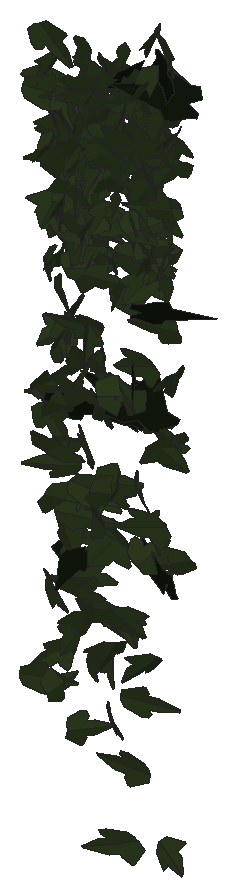
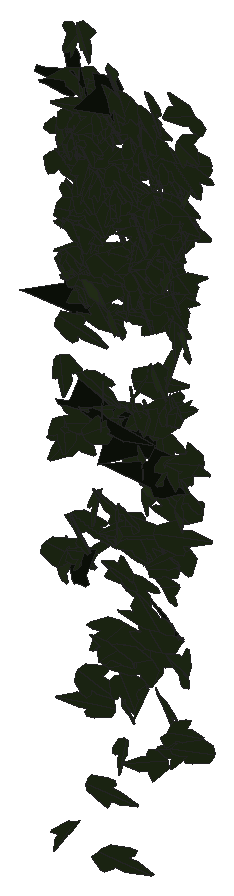
# SketchUp Ruby script. Lengths in millimetres.
U = 1.mm
M = Sketchup.active_model
def pt(a) = Geom::Point3d.new(a.map { |v| v * U })
def face(e, loops, mat)
  f = e.add_face(loops[0].map { |a| pt(a) })
  loops[1..].each { |l| e.add_face(l.map { |a| pt(a) }).erase! }
  f.material = f.back_material = mat if mat
  f
end
# faces: each face lists its corners as indices into pts; further lists are holes
def faces(e, pts, list, mat = nil) = list.each { |f| face(e, (f[0].is_a?(Array) ? f : [f]).map { |l| l.map { |i| pts[i] } }, mat) }
# xy, xz, yz: faces in a plane at the given z, y or x. An outline is a flat list of corners, or four numbers for a rectangle; further outlines are holes
def ring(l) = l.size == 4 ? [[l[0], l[1]], [l[2], l[1]], [l[2], l[3]], [l[0], l[3]]] : l.each_slice(2).to_a
def flat(e, list, mat, &to3) = list.each { |f| face(e, (f[0].is_a?(Array) ? f : [f]).map { |l| ring(l).map { |u, v| to3.(u, v) } }, mat) }
def xy(e, z, list, mat = nil) = flat(e, list, mat) { |x, y| [x, y, z] }
def xz(e, y, list, mat = nil) = flat(e, list, mat) { |x, z| [x, y, z] }
def yz(e, x, list, mat = nil) = flat(e, list, mat) { |y, z| [x, y, z] }
def lines(e, pts, list) = list.each { |a, b| e.add_line(pt(pts[a]), pt(pts[b])) }
# prism: a flat outline (further loops are holes) pulled along v
def prism(e, loops, v, mat = nil)
  f = face(e, loops, mat); d = Geom::Vector3d.new(v.map { |x| x * U })
  f.pushpull(f.normal.samedirection?(d) ? d.length : -d.length)
end
def box(e, o, s, mat = nil) = prism(e, [[o, [o[0] + s[0], o[1], o[2]], [o[0] + s[0], o[1] + s[1], o[2]], [o[0], o[1] + s[1], o[2]]]], [0, 0, s[2]], mat)
def at(x, y, z, deg = 0) = Geom::Transformation.translation(pt([x, y, z])) * Geom::Transformation.rotation(ORIGIN, Z_AXIS, deg.degrees)
def axes(o, x, y, z) = Geom::Transformation.new([*x, 0, *y, 0, *z, 0, *pt(o).to_a, 1])
def part(name) = M.definitions.add(name)
# library, detail: a bought-in or finely detailed component or shape, given as its bounding box
def library(name, o, s) = part(name).tap { |d| box(d.entities, o, s) }
def detail(e, o, s) = box(e.add_group.entities, o, s)
def put(e, d, t, mat = nil) = e.add_instance(d, t).tap { |i| i.material = mat if mat }
def group(e, t, mat = nil) = e.add_group.tap { |g| g.transformation = t; g.material = mat if mat }.entities
root = M.entities
M.materials.add("efeu1").color = [18, 25, 13]
M.materials.add("efeu2").color = [43, 57, 29]
c1 = part("ivyleaf_10")
p = [[0,12.8,-0.8],[-1.5,51.3,-10.9],[-4.9,51,-11.6],[-13.6,26.5,-7.3],[-13.2,15.9,-4.6],[-21.1,19.3,-7.2],
  [-29.5,16.3,-8.3],[-29.2,8.3,-6.2],[-19.7,-9.8,0.5],[-7.6,-13,4],[1,-12.2,5.8],[-0.4,51.1,-11.1],
  [-1.5,51.1,-10.9],[1,-12.4,5.9],[16.9,-12.4,3.5],[35.1,9.1,-5.1],[35,12.9,-6.1],[20.5,16.4,-4.9],
  [15.8,15,-3.8],[15.3,27.6,-7.1],[12.8,31.3,-7.8]]
faces(c1.entities,p,[[0,1,2,3,4,5,6,7,8,9,10],[11,12,0,13,14,15,16,17,18,19,20]],"efeu2")
c2 = part("ivyleaf_9")
p = [[39.1,54.8,31.7],[34.5,51.8,30.2],[-5.3,25.2,17.3],[-17.9,28.3,20.9],[-21.6,21.7,17],[-20.2,4.3,5.3],
  [-22.9,-0.3,2.5],[-17.1,-4,-0.6],[-2,-2.1,-1.2],[-0.7,-15.4,-10.1],[16.6,-22.3,-16.7],[21.1,-15.1,-12.5],
  [32.7,-10.7,-11],[46.1,-1.8,-6.6],[30.8,11.2,3.8]]
faces(c2.entities,p,[[0,1,2,3,4,5,6,7,8,9,10,11,12,13,14]],"efeu1")
put(root,c1,axes([1682.2,1042.4,971.2],[1.4117,-0.00868,-0.18926],[-0.36019,0.00139,-0.7418],[0.01667,0.76552,-0.0008]))
put(root,c1,axes([1675.2,1023.6,553.9],[0.05293,-0.25459,0.6538],[0.01552,0.65438,0.25447],[-1.33522,-0.00249,0.02887]))
put(root,c1,axes([1681.2,1038.1,1000.9],[0.03378,-0.57438,0.40168],[0.11995,-0.39887,-0.57315],[1.32855,0.05062,0.04154]))
put(root,c1,axes([1688,1047.7,186.4],[0.33561,0.25187,-0.58998],[-0.63511,-0.48655,-0.30745],[-1.0427,0.37742,-0.00263]))
put(root,c1,axes([1674.3,1055.3,499.6],[0.29859,-0.42722,0.47587],[0.48637,-0.40727,-0.44989],[1.11571,0.29188,0.06877]))
put(root,c1,axes([1678.9,1033.8,940.8],[-0.6045,0.61017,-0.04957],[0.04602,-0.0433,-0.68789],[-1.16419,-0.31854,-0.00145]))
put(root,c1,axes([1671.7,1043.4,720.8],[0.11818,-0.27819,-0.60931],[0.3396,-0.58294,0.28433],[-1.22872,-0.18787,0.01998]))
put(root,c1,axes([1685.7,1025.7,889.6],[-0.06636,-0.60794,-0.33331],[0.04395,0.33253,-0.60893],[1.31878,-0.04167,0.00352]))
put(root,c1,axes([1685.8,1035.2,810.1],[-0.53638,-0.5043,0.34703],[0.13496,-0.40636,-0.53293],[1.15723,-0.18635,0.223]))
put(root,c1,axes([1665.4,1020.3,154.4],[0.0195,-0.01031,0.67258],[0.80259,0.52415,0.00161],[-0.99738,0.42158,0.01444]))
put(root,c1,axes([1687.6,1044.1,627.9],[-0.29612,-0.09227,0.6372],[0.13498,-0.654,-0.07739],[1.2179,0.05005,0.1635]))
put(root,c1,axes([1684.7,1029.1,871.8],[-0.50878,0.64252,0.07306],[-0.04072,0.07022,-0.69587],[-1.23004,-0.26809,-0.00718]))
put(root,c1,axes([1696.8,1047.5,784.9],[-0.80236,-0.42863,0.25873],[-0.26192,-0.226,-0.59865],[0.91616,-0.44,0.05544]))
put(root,c1,axes([1704.1,1040.7,450.9],[-0.00229,-0.03494,0.72083],[-0.68178,-0.62573,-0.03093],[1.19235,-0.35786,-0.0163]))
put(root,c1,axes([1684.3,1043,888.6],[0.66874,0.5763,-0.05904],[-0.0603,-0.04983,-0.67497],[-1.1009,0.3528,0.00111]))
put(root,c1,axes([1693.3,1031.7,552],[-0.96734,-0.44501,-0.02178],[0.03135,0.01426,-0.67555],[0.84737,-0.50854,0.00012]))
put(root,c1,axes([1682.9,1039.4,789.4],[0.4895,0.60786,0.12352],[0.09127,0.11383,-0.66003],[-1.17698,0.26163,0.00018]))
put(root,c1,axes([1694.3,1028.4,878],[-0.90187,-0.52713,-0.06108],[0.07526,0.04658,-0.70881],[1.00713,-0.47551,-0.00173]))
put(root,c1,axes([1684,1051.8,800.7],[0.51563,-0.50543,0.32939],[0.44232,-0.24577,-0.56828],[1.05957,0.34857,0.07694]))
put(root,c1,axes([1695.7,1044.8,880.5],[-0.68389,-0.58029,0.05926],[0.03793,-0.08178,-0.67992],[1.10951,-0.35489,0.05977]))
put(root,c1,axes([1694.8,1034.5,742],[-0.04356,-0.62057,-0.32602],[0.03693,0.32551,-0.62095],[1.33362,-0.02928,0.00655]))
put(root,c1,axes([1671.4,1044.4,272.8],[-0.02481,-0.1435,0.7618],[1.20611,-0.44077,-0.07218],[0.84969,0.62147,0.12471]))
put(root,c1,axes([1694.2,1043.7,901.9],[-1.29705,-0.03436,-0.08463],[0.16956,-0.1094,-0.67297],[0.03837,-0.67798,0.11288]))
put(root,c1,axes([1702,1036.1,963.4],[-0.32402,-0.65447,0.15746],[-0.05188,-0.15558,-0.67614],[1.28008,-0.17197,0.01245]))
put(root,c1,axes([1675.9,1015.2,967.6],[0.12278,0.0972,0.73673],[0.96681,0.53396,-0.11493],[-1.03224,0.51168,-0.02002]))
put(root,c1,axes([1676.9,1034.9,516.8],[0.8799,-0.14543,0.57141],[1.02972,-0.18397,-0.48458],[0.44602,0.71162,-0.0085]))
put(root,c1,axes([1684.5,1045.6,629.5],[0.06756,-0.02653,-0.64087],[0.53277,-0.57686,0.03938],[-1.09836,-0.28144,-0.02031]))
put(root,c1,axes([1703.7,1025.7,693.8],[-0.62596,0.54085,0.3855],[-0.36541,0.33438,-0.63295],[-1.21008,-0.38075,-0.00828]))
put(root,c1,axes([1703.3,1018.7,617],[0.04614,0.02111,0.65659],[-0.43732,0.6158,-0.01132],[-1.17128,-0.22909,0.03009]))
put(root,c1,axes([1676.7,1029.1,1040.8],[0.8472,-0.1185,0.58486],[1.10503,-0.08248,-0.45863],[0.26224,0.73035,0.0431]))
put(root,c1,axes([1701.3,1039.4,918.7],[-1.20661,-0.26382,-0.0744],[0.21312,-0.07817,-0.67707],[0.47616,-0.63354,0.11452]))
put(root,c1,axes([1694.5,1021.2,147.4],[0.16088,0.20682,-0.66335],[0.53268,0.6015,0.2232],[1.21041,-0.2922,-0.01006]))
put(root,c1,axes([1697.7,1022.1,542.7],[-0.37693,-0.34664,-0.54634],[0.4934,0.48099,-0.39915],[1.12827,-0.32614,-0.00797]))
put(root,c1,axes([1706,1026,820.7],[0.09776,-0.61998,-0.28428],[0.07061,0.2872,-0.61965],[1.29615,0.03112,0.0552]))
put(root,c1,axes([1719.1,1014.5,930.3],[-0.01378,-0.03018,-0.71368],[-0.54088,0.65492,-0.02481],[1.24726,0.28368,-0.01865]))
put(root,c1,axes([1697.8,1056.1,630.8],[-0.11604,-0.02228,0.65518],[0.60424,-0.57669,0.00994],[1.09157,0.31686,0.06415]))
put(root,c1,axes([1694.8,1022.3,476],[-0.98786,-0.24058,0.41209],[0.70986,0.17523,0.57209],[-0.56645,0.63916,-0.00173]))
put(root,c1,axes([1704.5,1037.7,640.3],[0.48299,0.61188,-0.14748],[-0.10142,-0.13756,-0.66241],[-1.19357,0.25929,-0.00339]))
put(root,c1,axes([1710.4,1041.5,220.1],[0.78162,-0.58027,-0.08719],[-0.09644,0.07095,-0.7109],[1.1126,0.4138,-0.00037]))
put(root,c1,axes([1701.4,1047,822.5],[-0.4542,0.48237,-0.40974],[0.22277,-0.39671,-0.53521],[-1.18378,-0.25974,0.0565]))
put(root,c1,axes([1722.2,1025.2,746.4],[0.63081,-0.29587,0.60951],[-0.88776,0.39248,0.44417],[-0.93523,-0.57212,-0.01051]))
put(root,c1,axes([1710.9,1042.8,914],[1.28085,-0.10199,-0.12283],[-0.2173,0.06452,-0.67913],[0.21239,0.68107,0.04594]))
put(root,c1,axes([1716.2,1046.7,824.7],[-0.22251,-0.43206,0.49455],[-0.07021,-0.49722,-0.44311],[1.24787,-0.10502,0.06325]))
put(root,c1,axes([1700,1015.7,417],[-0.41381,-0.25233,-0.66481],[0.81433,0.50883,-0.33307],[1.08092,-0.47994,-0.00359]))
put(root,c1,axes([1725,1018.9,362.6],[0.79632,-0.23437,0.49683],[-0.84231,0.22615,0.4794],[-0.61934,-0.60891,-0.01319]))
put(root,c1,axes([1716.1,1045,675.4],[0.17895,-0.6424,0.03786],[0.00774,-0.03767,-0.64925],[1.22472,0.0941,-0.00143]))
put(root,c1,axes([1715.8,1037.2,903.1],[-0.33736,-0.63315,-0.1793],[0.11152,0.16977,-0.65742],[1.24743,-0.18641,0.01028]))
put(root,c2,axes([1719.9,1035.8,341],[-1.11083,0.21153,-0.47041],[0.8438,-0.15725,-0.62081],[-0.50163,-0.73295,-0.00257]))
put(root,c1,axes([1727.4,1024.5,571.5],[-1.20986,0.03884,0.16465],[-0.31338,0.00483,-0.63686],[-0.07387,-0.65666,0.00505]))
put(root,c1,axes([1722.8,1043.8,893.7],[-0.15376,-0.68139,0.05158],[-0.01385,-0.05107,-0.68616],[1.30045,-0.08111,-0.00121]))
put(root,c1,axes([1717.3,1038.8,826.6],[0.84804,0.48295,-0.15155],[-0.18425,-0.11686,-0.65706],[-0.94556,0.45592,-0.00788]))
put(root,c1,axes([1741.7,1037.8,653],[-0.26498,0.09197,-0.63195],[-1.18766,-0.15699,0.11463],[-0.25819,0.62777,0.12125]))
put(root,c1,axes([1718,1031.9,944.6],[0.92605,-0.49968,0.04922],[0.12628,-0.00395,-0.69602],[0.94722,0.48904,0.04467]))
put(root,c1,axes([1725.2,1032.4,960.3],[-1.11796,0.36009,0.06976],[-0.15366,0.00153,-0.6878],[-0.68094,-0.59154,0.04068]))
put(root,c1,axes([1725.4,1039.2,594.2],[-0.58591,-0.56385,-0.32507],[-0.273,-0.29198,0.64229],[-1.20823,0.3394,0.01251]))
put(root,c2,axes([1695.9,1036.3,531.8],[0.72028,0.06599,0.67345],[1.25803,0.12905,-0.38411],[-0.27557,0.76165,0.00673]))
put(root,c1,axes([1718.4,1026.6,965],[0.76789,0.56481,-0.00031],[-0.0004,-0.00023,-0.69412],[-1.07495,0.40347,0.00003]))
put(root,c1,axes([1730.5,1036.3,970],[-0.43937,-0.65579,0.11632],[-0.04033,-0.11582,-0.695],[1.26695,-0.23111,0.01822]))
put(root,c1,axes([1727.8,1028.1,888.6],[0.89452,-0.48559,-0.08372],[-0.10961,0.06076,-0.6758],[0.93139,0.47352,0.00087]))
put(root,c1,axes([1728.9,1038,875.7],[0.111,-0.66018,0.16754],[0.04542,-0.16606,-0.66269],[1.29548,0.06239,0.00888]))
put(root,c1,axes([1732,1030.2,971.7],[-0.84229,-0.55487,-0.0039],[0.02687,-0.00627,-0.7096],[1.05572,-0.44254,0.01495]))
put(root,c1,axes([1715.2,1040.8,940.9],[0.27115,-0.37329,0.56187],[0.74397,-0.42233,-0.3797],[1.0463,0.39703,0.12437]))
put(root,c1,axes([1723.9,1035.3,841.5],[-0.10306,0.4966,-0.4529],[-0.0036,-0.45448,-0.49811],[-1.27916,-0.03873,0.03789]))
put(root,c1,axes([1731.1,1015.9,943.2],[0.11586,0.01636,-0.71351],[-0.00247,0.7161,0.01631],[1.35831,-0.00009,0.06089]))
put(root,c1,axes([1713.8,1047.1,767],[-0.60718,0.36771,-0.58844],[0.75547,-0.4345,-0.48673],[-1.08316,-0.50917,-0.00962]))
put(root,c1,axes([1739.8,1046.8,802.5],[-0.79337,-0.36812,0.37167],[-0.20147,-0.40606,-0.5209],[0.975,-0.38345,0.1948]))
put(root,c1,axes([1726,1030.1,288.2],[-1.09927,-0.19976,0.23763],[0.42547,0.08061,0.61115],[-0.40993,0.61934,-0.0029]))
put(root,c1,axes([1726.3,1026.6,847.5],[-1.15604,-0.2101,-0.29813],[0.55323,0.07091,-0.64222],[0.41923,-0.67291,0.02541]))
put(root,c1,axes([1734.4,1031.5,984.3],[-1.28812,0.14275,-0.03308],[0.06272,-0.00407,-0.6917],[-0.27173,-0.67761,-0.00281]))
put(root,c1,axes([1722.1,1041,852.1],[1.25294,-0.03637,0.27245],[0.51977,0.00655,-0.65904],[0.05919,0.71245,0.01997]))
put(root,c1,axes([1742.1,1025.6,1037.9],[0.61553,-0.54059,-0.35961],[-0.24038,0.3417,-0.62725],[1.21209,0.34229,0.05822]))
put(root,c1,axes([1740.6,1025.6,262.7],[-0.55972,-0.58216,-0.07966],[0.06972,0.07074,-0.65223],[1.11611,-0.29637,0.00079]))
put(root,c1,axes([1750,1022.2,487.7],[-0.03905,0.28492,-0.66438],[-0.42548,0.62956,0.27689],[1.30837,0.21324,0.07022]))
put(root,c1,axes([1733.4,1026.9,583.3],[0.37885,-0.67643,-0.07018],[0.07262,-0.0619,0.70486],[-1.29226,-0.20179,0.01903]))
put(root,c1,axes([1728.9,1034,315.5],[1.4185,-0.09526,-0.21151],[0.4012,-0.01895,0.75135],[-0.18427,-0.77452,0.00763]))
put(root,c1,axes([1742.1,1038.8,756.2],[0.4977,-0.60075,0.07958],[0.11279,-0.06091,-0.65452],[1.1478,0.26648,0.02981]))
put(root,c1,axes([1745.6,1035.5,982],[0.36573,-0.68006,-0.0418],[0.01402,0.0455,-0.70642],[1.29665,0.19132,0.01943]))
put(root,c1,axes([1757,1037.8,546.9],[-0.75474,0.33601,0.42889],[-0.69484,0.22987,-0.51767],[-0.76969,-0.537,0.04677]))
put(root,c1,axes([1749.5,1040.5,872.6],[0.41,-0.62278,-0.24174],[-0.14533,0.22938,-0.65898],[1.2631,0.22854,0.00265]))
put(root,c1,axes([1747.4,1041.3,875],[1.15809,-0.25398,-0.12296],[-0.19938,0.06807,-0.659],[0.49867,0.61705,0.02209]))
put(root,c1,axes([1741.2,1036.8,863],[0.80139,0.52899,-0.03109],[-0.04033,-0.02287,-0.67611],[-1.00771,0.4216,0.00233]))
put(root,c1,axes([1745.7,1035.6,423.3],[1.02435,0.37125,-0.16576],[-0.26335,-0.09132,-0.65384],[-0.7276,0.55572,0.00329]))
put(root,c1,axes([1725.5,1026,735.9],[0.36837,-0.00511,-0.67426],[1.10532,0.35766,0.164],[0.65199,-0.60346,0.10291]))
put(root,c1,axes([1741.5,1037.7,996.4],[0.84769,-0.53247,0.01746],[0.26458,0.09419,-0.67381],[0.97881,0.43568,0.16701]))
put(root,c1,axes([1749.5,1024.7,806.4],[0.24073,-0.66773,-0.03536],[-0.00199,0.03578,-0.67958],[1.2726,0.12637,0.00562]))
put(root,c1,axes([1744.1,1027.9,780.7],[1.22202,-0.03248,-0.01708],[-0.03263,-0.0008,-0.64291],[0.06176,0.64232,-0.00167]))
put(root,c1,axes([1719.6,1022.1,396.8],[0.2159,-0.10818,-0.72291],[1.38833,-0.02992,0.11895],[-0.08876,-0.73114,0.1021]))
put(root,c1,axes([1745.6,1030.4,651.8],[-0.01198,0.59882,-0.47127],[-0.0974,-0.47056,-0.59723],[-1.44701,0.02672,0.0441]))
put(root,c1,axes([1748.5,1027.6,779.4],[-1.25098,0.11246,-0.06956],[0.12921,-0.01563,-0.66684],[-0.21596,-0.66079,0.00394]))
put(root,c1,axes([1765.4,1026.9,1013.9],[-1.15451,0.13389,0.36427],[-0.72583,-0.08032,-0.60557],[-0.13696,-0.70301,0.13856]))
put(root,c1,axes([1754.8,1030.7,975.5],[-0.69442,-0.59555,0.12564],[-0.03488,-0.13567,-0.69631],[1.15786,-0.36126,0.05437]))
put(root,c1,axes([1754.8,1022.6,203.7],[-0.22821,0.37286,0.53038],[-0.38068,0.49179,-0.39096],[-1.17371,-0.232,0.02367]))
put(root,c1,axes([1738.2,1012.1,112.2],[-0.01725,-0.01678,-0.70201],[0.84865,0.54222,-0.01871],[1.03242,-0.44598,0.00366]))
put(root,c1,axes([1744.2,1038.7,603.6],[-0.71152,0.46001,-0.27352],[0.34266,-0.2061,-0.5927],[-0.95919,-0.41486,-0.00884]))
put(root,c1,axes([1756.2,1027.8,999.2],[-1.10254,-0.38426,-0.03726],[0.05715,0.02214,-0.69517],[0.73254,-0.58008,-0.00184]))
put(root,c1,axes([1751.7,1034.8,810.3],[0.63258,0.55106,-0.23253],[-0.22239,-0.20107,-0.64353],[-1.11638,0.3523,-0.00356]))
put(root,c1,axes([1756.7,1035,874.5],[0.63676,0.53734,-0.24738],[-0.39367,-0.15999,-0.62729],[-1.05477,0.38411,0.08478]))
put(root,c1,axes([1750.8,1038.3,867.2],[1.39893,0.06993,-0.02019],[-0.03968,0.00595,-0.73832],[-0.13272,0.73529,0.00789]))
put(root,c1,axes([1734.6,1023.3,807.6],[-0.74303,-0.02275,-0.61158],[1.16132,0.04119,-0.39106],[0.08936,-0.7244,-0.00303]))
put(root,c1,axes([1739.6,1045.9,266.5],[-0.99445,0.1784,-0.50215],[0.89598,-0.17499,-0.55204],[-0.47523,-0.70324,0.00998]))
put(root,c1,axes([1774,1026.3,906.5],[-1.01754,-0.07883,0.42758],[-0.76533,-0.16803,-0.5338],[0.31464,-0.66365,0.08436]))
put(root,c1,axes([1752.6,1038.2,842.2],[0.17788,-0.63292,-0.20987],[0.3262,0.22761,-0.61007],[1.22643,0.03126,0.1927]))
put(root,c1,axes([1736.9,1028.3,437],[0.37935,0.20882,0.65979],[0.90115,0.4596,-0.28851],[-0.96057,0.51364,-0.01009]))
put(root,c1,axes([1774.3,1011.8,406.3],[0.01022,-0.03455,-0.71906],[-0.66102,0.62973,-0.03285],[1.20008,0.34716,-0.01197]))
put(root,c1,axes([1770.6,1037,764.9],[-0.58672,0.50594,0.23881],[-0.42246,0.13967,-0.58246],[-0.97738,-0.36409,0.10841]))
put(root,c1,axes([1771,1040.4,223.3],[-0.4605,-0.66163,0.09856],[-0.06697,-0.09208,-0.70448],[1.27135,-0.2445,-0.00141]))
put(root,c1,axes([1751.8,1041.3,614.4],[0.54256,-0.28805,0.53632],[0.73765,-0.37081,-0.40517],[0.89348,0.48105,0.00883]))
put(root,c1,axes([1769.7,1033.3,366.5],[1.31035,-0.08443,-0.21605],[-0.40793,0.02718,-0.69366],[0.1688,0.72109,0.00085]))
put(root,c1,axes([1757.2,1042.6,800.5],[0.69305,-0.37085,0.47842],[0.66331,-0.32804,-0.51956],[0.94194,0.50387,0.01387]))
put(root,c1,axes([1773.5,1033.6,826],[0.56721,0.47466,-0.40116],[-0.43846,-0.32883,-0.56022],[-1.09852,0.37633,0.01647]))
put(root,c1,axes([1777.8,1033.2,129.6],[-0.67409,0.45141,0.33193],[-0.39653,0.25843,-0.57377],[-0.98993,-0.41091,0.0038]))
put(root,c1,axes([1767.5,1017.3,950.3],[0.13443,-0.07207,0.71549],[0.01923,0.71896,0.07142],[-1.36847,0.00303,0.07129]))
put(root,c1,axes([1759.5,1050,201.4],[0.51509,-0.32237,0.5824],[0.77825,-0.41558,-0.42005],[0.99968,0.48963,0.02692]))
put(root,c1,axes([1779.2,1025.2,940.1],[-1.30708,-0.01609,0.06992],[-0.13284,-0.00574,-0.68696],[0.03157,-0.69031,0.00408]))
put(root,c1,axes([1773.1,1039.5,903.9],[-0.32668,-0.63889,-0.1522],[0.22182,0.12518,-0.65693],[1.23013,-0.19224,0.07804]))
put(root,c1,axes([1761.4,1013.1,741.6],[-0.46118,-0.2459,-0.64819],[0.84029,0.47465,-0.34512],[1.01724,-0.50357,-0.00878]))
put(root,c2,axes([1762.2,1027,568.8],[1.42618,0.1265,-0.10238],[-0.19214,-0.01703,-0.75996],[-0.24293,0.75613,0.00002]))
put(root,c1,axes([1774.6,1032,1026.4],[-1.04485,0.43286,-0.04095],[0.02463,-0.04966,-0.69843],[-0.82713,-0.54828,0.03093]))
put(root,c1,axes([1762.3,1025,440.6],[-0.23005,-0.15799,-0.70736],[0.83752,0.55382,-0.19889],[1.09605,-0.45634,0.00351]))
put(root,c1,axes([1779.8,1038.2,929.4],[-0.55048,-0.63808,0.02152],[0.02618,-0.02984,-0.70014],[1.21481,-0.2885,0.02484]))
put(root,c1,axes([1787.1,1031.3,819.1],[1.11631,0.00229,-0.36569],[-0.69584,0.01815,-0.58631],[0.01458,0.69096,0.01661]))
put(root,c1,axes([1784.5,1030.5,450.2],[0.00093,-0.50295,-0.54014],[-0.01138,0.54012,-0.50294],[1.4046,0.00471,-0.00372]))
put(root,c1,axes([1758.5,1047.1,376.5],[0.13444,-0.00515,0.66044],[1.18714,-0.21782,-0.06842],[0.41319,0.62748,-0.01832]))
put(root,c1,axes([1806.5,1032.4,922],[-0.41513,-0.00911,0.66246],[-1.19284,-0.22322,-0.20944],[0.4087,-0.66076,0.06162]))
put(root,c1,axes([1795.3,1050.6,806.9],[-0.71333,-0.34136,0.4119],[-0.48945,-0.32603,-0.50422],[0.89278,-0.45149,0.05268]))
put(root,c1,axes([1800.7,1031.7,-32.3],[0.59671,0.13446,-0.61128],[-1.11169,-0.18273,-0.33979],[-0.42789,0.66225,0.03036]))
put(root,c1,axes([1789.9,1024.8,977.6],[0.85083,-0.50313,-0.2244],[-0.29331,0.16323,-0.67302],[1.00661,0.47283,-0.00643]))
put(root,c1,axes([1809.5,1043.3,65.2],[0.10487,-0.03845,-0.6607],[-1.19109,0.21262,-0.06457],[0.40969,0.62798,-0.0186]))
put(root,c1,axes([1790.9,1025.1,845.9],[0.42103,-0.60992,-0.14111],[-0.03686,0.14293,-0.64811],[1.19089,0.22005,0.02983]))
put(root,c1,axes([1788.6,1039.2,727.9],[0.1931,-0.62963,0.21567],[0.14335,-0.20589,-0.63653],[1.25852,0.12006,0.03941]))
put(root,c2,axes([1819.1,1035.8,569.4],[-1.01489,-0.03605,-0.56706],[-1.05801,-0.12779,0.5309],[-0.22373,0.76784,0.06173]))
put(root,c1,axes([1787.5,1020.9,881.6],[-0.45904,-0.49257,-0.46586],[0.37304,0.42269,-0.5484],[1.23522,-0.3107,-0.00751]))
put(root,c1,axes([1766.2,1039.5,447.3],[0.58113,-0.27764,-0.64369],[1.04524,-0.3416,0.40786],[-0.82916,-0.62521,0.06301]))
put(root,c1,axes([1778.2,1048.1,266.1],[1.0532,-0.06363,0.36928],[0.69502,-0.05604,-0.55691],[0.15984,0.66292,-0.01163]))
put(root,c1,axes([1791.2,1041.3,914],[1.13712,-0.32328,0.03595],[0.06794,-0.00956,-0.67927],[0.61532,0.59848,0.00857]))
put(root,c1,axes([1787.6,1032.9,907.2],[1.15593,-0.27379,0.16454],[0.32063,-0.02577,-0.66474],[0.51651,0.62872,0.04441]))
put(root,c1,axes([1800.7,1027.7,1052.4],[0.52766,-0.66783,-0.04679],[-0.0291,0.04431,-0.72308],[1.27379,0.27766,0.00286]))
put(root,c1,axes([1791.7,1023.9,283.1],[-1.07634,-0.28096,-0.38375],[0.63801,0.18747,-0.63128],[0.64211,-0.65724,-0.01602]))
put(root,c1,axes([1807.9,1053.4,564.3],[0.04575,0.2892,0.67807],[-0.13468,-0.6744,0.29014],[1.3965,-0.07451,0.00577]))
put(root,c1,axes([1807.1,1035.3,995.9],[-0.30834,-0.67993,0.11129],[0.00049,-0.11439,-0.69846],[1.31126,-0.15984,0.02643]))
put(root,c1,axes([1802.9,1034.6,1028.4],[-1.20064,0.3128,-0.09955],[0.08841,-0.12842,-0.69791],[-0.61845,-0.62562,0.09349]))
put(root,c1,axes([1808.3,1031.7,999.7],[-1.11277,0.38831,0.11251],[-0.21142,0.0359,-0.70119],[-0.73981,-0.59433,0.03116]))
put(root,c1,axes([1806.4,1018.8,988.8],[0.39058,-0.61376,-0.3124],[0.04192,0.33166,-0.63713],[1.31004,0.17238,0.11353]))
put(root,c1,axes([1820.4,1017.9,582.6],[0.78946,-0.11474,0.54991],[-0.99214,0.17609,0.42996],[-0.39837,-0.66593,0.01895]))
put(root,c1,axes([1786.1,1014.6,585.5],[0.30987,-0.1407,-0.73673],[1.10704,0.49964,0.03313],[0.90122,-0.56537,0.21262]))
put(root,c1,axes([1790.1,1036.7,978.8],[0.65743,-0.39762,-0.46848],[0.61006,-0.34191,0.52654],[-0.99774,-0.47106,0.01326]))
put(root,c2,axes([1797.9,1021.7,1021.1],[0.45827,0.34365,0.64076],[0.75252,0.50457,-0.41919],[-1.16131,0.46256,-0.01878]))
put(root,c1,axes([1809.8,1028.8,1014],[-1.25532,0.28506,-0.00532],[0.00368,-0.00894,-0.71851],[-0.54262,-0.65954,0.00744]))
put(root,c1,axes([1823.4,1039.1,628.8],[0.75715,-0.14512,-0.48941],[-0.82411,0.23265,-0.42098],[0.51449,0.58623,0.04592]))
put(root,c1,axes([1799.8,1034.8,706.6],[1.26434,-0.11572,-0.11217],[0.22324,0.02094,0.67313],[-0.21032,-0.6734,0.0402]))
put(root,c2,axes([1819.1,1020.7,614],[0.23516,-0.06211,-0.76596],[-1.19473,0.43933,-0.13689],[0.84362,0.63949,0.01965]))
put(root,c1,axes([1807.6,1031,952.2],[-1.20817,0.21978,-0.15697],[0.27913,-0.05616,-0.67176],[-0.43162,-0.65151,0.00495]))
put(root,c1,axes([1824.1,1039.2,868.8],[-1.18618,-0.0477,0.26578],[-0.49702,-0.0635,-0.6238],[0.13065,-0.67458,0.03993]))
put(root,c1,axes([1821.1,1029.8,461],[-0.56438,0.42219,0.45509],[-0.4841,0.37743,-0.51589],[-1.07771,-0.39063,-0.00659]))
put(root,c1,axes([1822.8,1048.6,217.6],[-0.21349,-0.53913,0.45324],[-0.23213,-0.43715,-0.55018],[1.32025,-0.16404,-0.02345]))
put(root,c1,axes([1806.5,1048.2,754.1],[-0.1685,-0.45137,-0.44245],[0.25239,-0.45009,0.43263],[-1.17616,-0.03192,0.15622]))
put(root,c1,axes([1805.3,1036.8,1000.9],[-0.70633,-0.35946,-0.48251],[0.71048,0.30704,-0.51587],[0.89807,-0.52562,0.02863]))
put(root,c1,axes([1821.7,1026.5,801.5],[-0.98392,0.35185,0.17256],[-0.26313,0.10353,-0.62531],[-0.69787,-0.5351,-0.00752]))
put(root,c1,axes([1814.5,1046.3,912],[-0.82404,0.49382,-0.19017],[0.12276,-0.19463,-0.65226],[-0.99961,-0.43099,0.07667]))
put(root,c1,axes([1793.9,1040.6,770.1],[-0.23192,-0.03802,-0.69789],[1.3118,0.11084,-0.12639],[0.2204,-0.69972,0.0179]))
put(root,c1,axes([1815.5,1029.2,834.3],[-0.23435,0.68542,0.03123],[-0.01884,0.02995,-0.69638],[-1.3057,-0.12345,0.00444]))
put(root,c1,axes([1824.6,1041.4,900.5],[-0.64708,-0.5928,0.00312],[-0.01921,0.0022,-0.68331],[1.12806,-0.34,-0.00985]))
put(root,c1,axes([1828,1036.8,746.2],[0.79278,0.3968,-0.3783],[-0.55124,-0.24411,-0.57497],[-0.88589,0.50699,0.01924]))
put(root,c1,axes([1829.9,1039.1,879.4],[-0.51108,-0.56151,0.25077],[-0.13001,-0.24471,-0.62109],[1.16316,-0.27407,0.04077]))
put(root,c1,axes([1824.4,1037.7,909.4],[-0.36851,0.62062,0.25663],[-0.18813,0.23784,-0.64975],[-1.26424,-0.2163,0.02188]))
put(root,c1,axes([1826.5,1033,985.6],[-1.01174,-0.47405,0.02236],[0.15884,-0.12644,-0.69633],[0.88914,-0.51683,0.14984]))
put(root,c1,axes([1832.3,1029.9,929.5],[-1.16796,-0.27764,0.07523],[-0.06193,-0.10912,-0.66812],[0.54394,-0.60857,0.08547]))
put(root,c1,axes([1826.2,1039.9,923.2],[-0.50487,-0.5787,-0.25013],[0.29235,0.20386,-0.63456],[1.1637,-0.30228,0.0509]))
put(root,c1,axes([1846.7,1028.9,420.1],[0.75297,-0.12717,-0.55307],[-1.01171,0.153,-0.41544],[0.37815,0.66257,-0.01022]))
put(root,c2,axes([1827.6,1021.5,567],[-1.23333,0.06814,0.51258],[0.95493,-0.11585,0.64973],[0.23795,0.81808,0.04932]))
put(root,c1,axes([1834.9,1056.6,771.8],[-0.37832,0.22652,0.58226],[0.05555,-0.60699,0.2461],[1.18776,0.10054,0.17395]))
put(root,c1,axes([1813.1,1036.6,1006.3],[-0.0228,-0.03667,0.70751],[0.91393,0.51984,0.03507],[-0.99134,0.48009,0.01606]))
put(root,c1,axes([1835.5,1026.7,1025.3],[-0.04525,-0.65358,-0.27372],[0.12817,0.27055,-0.65186],[1.34246,-0.04786,0.05301]))
put(root,c1,axes([1834.7,1024.5,841.1],[-0.19115,0.55451,0.38958],[-0.18741,0.37772,-0.56301],[-1.27608,-0.13853,0.02433]))
put(root,c1,axes([1814,1028.2,170.9],[0.06051,-0.06086,0.66522],[0.99585,0.41626,0.01307],[-0.7903,0.51986,0.06741]))
put(root,c1,axes([1856.8,1043.7,854.7],[0.18038,0.07272,-0.66694],[-1.18708,-0.23852,-0.11465],[-0.47025,0.63,0.03358]))
put(root,c1,axes([1861.6,1037.4,692.3],[-0.3428,0.04238,0.65889],[-1.24751,-0.09347,-0.17317],[0.15085,-0.67664,0.06519]))
put(root,c1,axes([1834.4,1041,777.9],[1.19399,-0.16316,0.01158],[0.02053,-0.00451,-0.64823],[0.31064,0.62745,-0.00165]))
put(root,c1,axes([1823.8,1051.4,401.9],[0.37016,-0.35192,-0.5134],[0.49975,-0.44129,0.40196],[-1.07405,-0.32661,0.01009]))
put(root,c1,axes([1839.9,1040.9,959.8],[1.13742,-0.33867,-0.11277],[-0.16226,0.07812,-0.68645],[0.65968,0.60314,0.02559]))
put(root,c1,axes([1822.3,1020.3,823],[0.49424,0.18711,-0.62084],[0.91197,0.39519,0.31954],[0.83142,-0.5447,0.01857]))
put(root,c1,axes([1849.3,1044.9,792.5],[-0.60595,-0.45924,0.38935],[-0.2682,-0.37136,-0.55326],[1.11404,-0.33919,0.07858]))
put(root,c1,axes([1833.9,1020.9,372.8],[0.47648,0.24696,-0.67012],[0.53404,0.61898,0.33294],[1.24992,-0.35861,0.1132]))
put(root,c1,axes([1839.8,1046.7,834.9],[1.23546,-0.12838,-0.01838],[-0.03399,0.00443,-0.66172],[0.24448,0.64939,0.00088]))
put(root,c1,axes([1844.7,1019.5,792.9],[-0.00319,-0.56962,-0.38031],[0.10461,0.37898,-0.56786],[1.29933,-0.03191,0.04479]))
put(root,c1,axes([1854.6,1037.5,759.7],[0.67342,-0.33254,-0.46485],[-0.47209,0.4032,-0.47725],[0.97998,0.42275,0.08952]))
put(root,c1,axes([1847.9,1027,1098.2],[0.17499,-0.71424,-0.05387],[0.00802,0.05485,-0.72005],[1.36319,0.09137,0.01115]))
put(root,c1,axes([1851.4,1026.4,946.1],[-0.91311,-0.51467,0.0466],[-0.05523,-0.03666,-0.7036],[0.98197,-0.48064,0.00376]))
put(root,c1,axes([1839.4,1031.8,802.7],[0.66905,0.60451,0.06889],[0.06616,0.05947,-0.69929],[-1.15605,0.35326,-0.00015]))
put(root,c1,axes([1853.7,1042.3,793.8],[-0.27683,-0.55469,0.3004],[-0.13387,-0.2921,-0.57342],[1.19307,-0.16148,0.00536]))
put(root,c2,axes([1863.1,1026.5,345.2],[0.28822,-0.35778,0.66963],[-0.28746,0.65497,0.38411],[-1.41606,-0.20578,0.05832]))
put(root,c1,axes([1835.7,1033.2,560.3],[-0.74575,0.14245,-0.49831],[0.85555,-0.21748,-0.41566],[-0.49089,-0.59544,0.0326]))
put(root,c1,axes([1849.9,1031.2,1042.5],[0.82114,0.56179,-0.0689],[-0.17524,-0.01581,-0.70553],[-1.06285,0.43663,0.0631]))
put(root,c1,axes([1872.9,1020.4,866.1],[-0.48317,0.29947,0.56995],[-1.10173,0.162,-0.34297],[-0.53637,-0.60253,0.19106]))
put(root,c1,axes([1857.1,1032.6,983],[-0.5654,-0.63648,0.12707],[0.01679,-0.1437,-0.69913],[1.23514,-0.2894,0.06768]))
put(root,c1,axes([1855.5,1036.1,969.7],[0.54217,-0.61924,-0.18683],[0.00423,0.20508,-0.67635],[1.23101,0.27203,0.08461]))
put(root,c1,axes([1852,1052.5,781.3],[0.18304,-0.31245,0.57498],[0.29668,-0.55349,-0.32685],[1.20959,0.18304,-0.00684]))
put(root,c1,axes([1874.5,1043.3,376],[-0.4412,-0.23583,0.59657],[-0.76128,-0.44277,-0.33047],[0.95447,-0.46216,0.01219]))
put(root,c2,axes([1874,1016.3,1058],[0.15071,-0.01037,-0.77865],[-1.41326,0.23468,-0.07864],[0.44629,0.74665,0.01391]))
put(root,c1,axes([1870.2,1038.9,920.8],[-0.72434,-0.496,0.29972],[-0.2511,-0.27501,-0.62262],[1.07399,-0.39881,0.05658]))
put(root,c2,axes([1891.8,1030.3,1018.8],[-0.93301,0.07444,0.60663],[-1.14916,0.0615,-0.49549],[-0.18022,-0.77753,0.01889]))
put(root,c1,axes([1865.7,1033.7,959.9],[-1.18639,0.28816,0.08014],[-0.14022,0.03162,-0.68674],[-0.5517,-0.6277,0.0022]))
put(root,c1,axes([1864,1030.7,946.9],[0.85519,-0.52861,-0.02147],[-0.025,0.01702,-0.69379],[1.00657,0.44954,0.00101]))
put(root,c1,axes([1864.6,1024.4,950.9],[-0.32662,0.65159,0.18226],[-0.16879,0.16474,-0.67248],[-1.27659,-0.18849,0.04229]))
put(root,c1,axes([1857.1,1052.7,359.1],[0.09228,-0.19011,0.65797],[0.54282,-0.5941,-0.19267],[1.18507,0.28693,0.03702]))
put(root,c1,axes([1868.8,1037,960.5],[-0.02845,-0.6986,-0.082],[-0.01837,0.08221,-0.69867],[1.33858,-0.01372,-0.01133]))
put(root,c1,axes([1860,1027.8,1089.7],[-0.61651,0.59208,-0.24043],[0.16234,-0.22708,-0.67414],[-1.20533,-0.33342,0.03218]))
put(root,c1,axes([1859.3,1031.6,852],[-0.24325,0.65961,-0.33241],[0.13489,-0.32484,-0.67184],[-1.39928,-0.14598,-0.00698]))
put(root,c1,axes([1860,1028.2,529.4],[-0.76401,-0.45576,-0.39586],[0.59662,0.24889,-0.60444],[0.98186,-0.50587,0.05926]))
put(root,c1,axes([1869.5,1032.1,545.4],[-0.51406,-0.61457,-0.11926],[0.09838,0.10755,-0.6713],[1.1874,-0.27498,0.00399]))
put(root,c1,axes([1870.2,1036.5,631.6],[-0.16529,-0.7106,-0.1792],[0.06967,0.17602,-0.71574],[1.39301,-0.09312,0.01453]))
put(root,c2,axes([1843,1013.6,719.3],[0.82887,0.06376,0.62922],[1.12505,0.23053,-0.43252],[-0.42786,0.72969,0.08166]))
put(root,c1,axes([1865.4,1026.5,-16.2],[0.04516,0.66502,0.25191],[0.02361,0.25162,-0.66543],[-1.35322,0.02658,-0.0032]))
